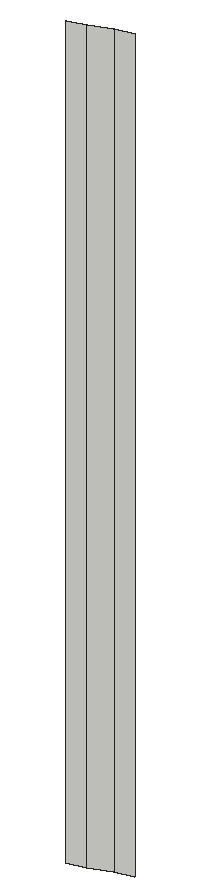
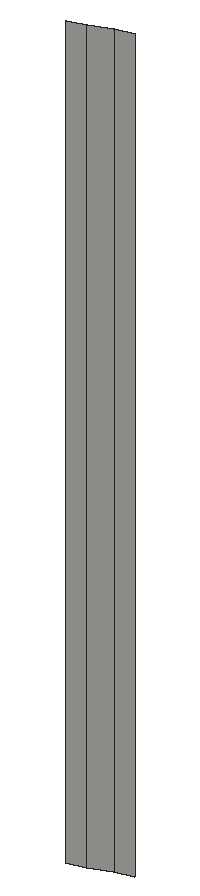
# SketchUp Ruby script. Lengths in inches.
U = 1.inch
M = Sketchup.active_model
def pt(a) = Geom::Point3d.new(a.map { |v| v * U })
def face(e, loops, mat)
  f = e.add_face(loops[0].map { |a| pt(a) })
  loops[1..].each { |l| e.add_face(l.map { |a| pt(a) }).erase! }
  f.material = f.back_material = mat if mat
  f
end
# faces: each face lists its corners as indices into pts; further lists are holes
def faces(e, pts, list, mat = nil) = list.each { |f| face(e, (f[0].is_a?(Array) ? f : [f]).map { |l| l.map { |i| pts[i] } }, mat) }
# xy, xz, yz: faces in a plane at the given z, y or x. An outline is a flat list of corners, or four numbers for a rectangle; further outlines are holes
def ring(l) = l.size == 4 ? [[l[0], l[1]], [l[2], l[1]], [l[2], l[3]], [l[0], l[3]]] : l.each_slice(2).to_a
def flat(e, list, mat, &to3) = list.each { |f| face(e, (f[0].is_a?(Array) ? f : [f]).map { |l| ring(l).map { |u, v| to3.(u, v) } }, mat) }
def xy(e, z, list, mat = nil) = flat(e, list, mat) { |x, y| [x, y, z] }
def xz(e, y, list, mat = nil) = flat(e, list, mat) { |x, z| [x, y, z] }
def yz(e, x, list, mat = nil) = flat(e, list, mat) { |y, z| [x, y, z] }
def lines(e, pts, list) = list.each { |a, b| e.add_line(pt(pts[a]), pt(pts[b])) }
# prism: a flat outline (further loops are holes) pulled along v
def prism(e, loops, v, mat = nil)
  f = face(e, loops, mat); d = Geom::Vector3d.new(v.map { |x| x * U })
  f.pushpull(f.normal.samedirection?(d) ? d.length : -d.length)
end
def box(e, o, s, mat = nil) = prism(e, [[o, [o[0] + s[0], o[1], o[2]], [o[0] + s[0], o[1] + s[1], o[2]], [o[0], o[1] + s[1], o[2]]]], [0, 0, s[2]], mat)
def at(x, y, z, deg = 0) = Geom::Transformation.translation(pt([x, y, z])) * Geom::Transformation.rotation(ORIGIN, Z_AXIS, deg.degrees)
def axes(o, x, y, z) = Geom::Transformation.new([*x, 0, *y, 0, *z, 0, *pt(o).to_a, 1])
def part(name) = M.definitions.add(name)
# library, detail: a bought-in or finely detailed component or shape, given as its bounding box
def library(name, o, s) = part(name).tap { |d| box(d.entities, o, s) }
def detail(e, o, s) = box(e.add_group.entities, o, s)
def put(e, d, t, mat = nil) = e.add_instance(d, t).tap { |i| i.material = mat if mat }
def group(e, t, mat = nil) = e.add_group.tap { |g| g.transformation = t; g.material = mat if mat }.entities
root = M.entities
p = [[215.28,317.13,231],[215.21,317.11,231],[215.21,317.11,234],[215.28,317.13,234],[215.36,317.16,231],[215.36,317.16,234],
  [215.43,317.18,231],[215.43,317.18,234]]
faces(root,p,[[0,1,2,3],[4,0,3,5],[6,4,5,7]])
